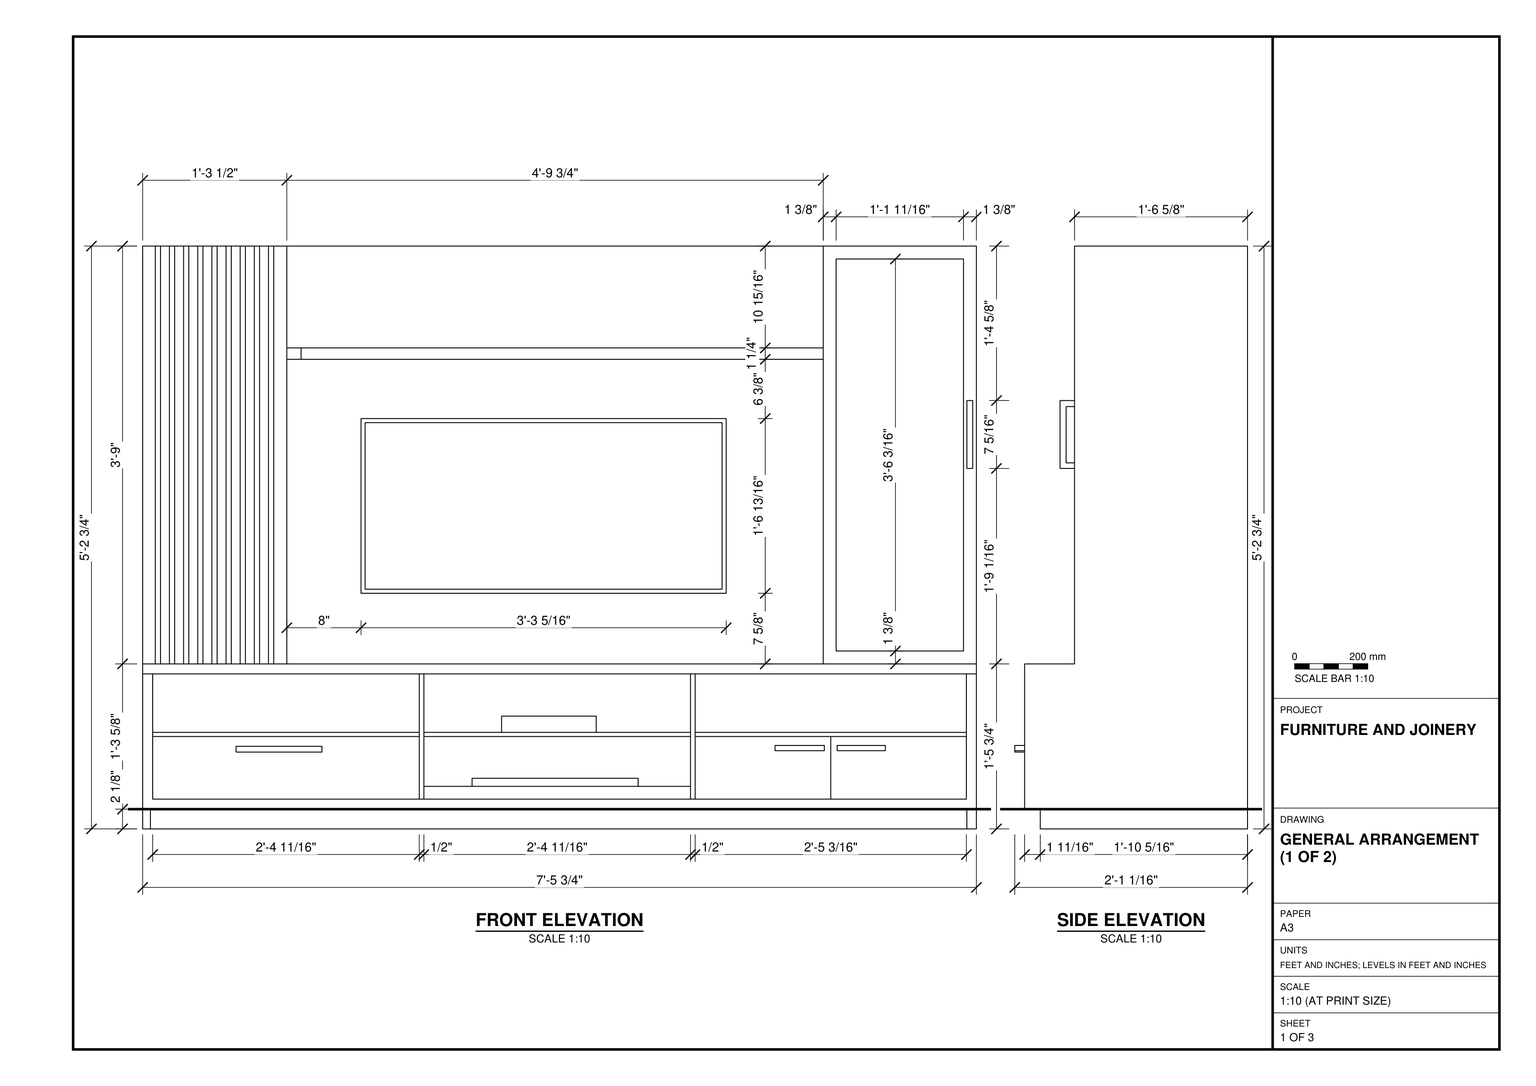
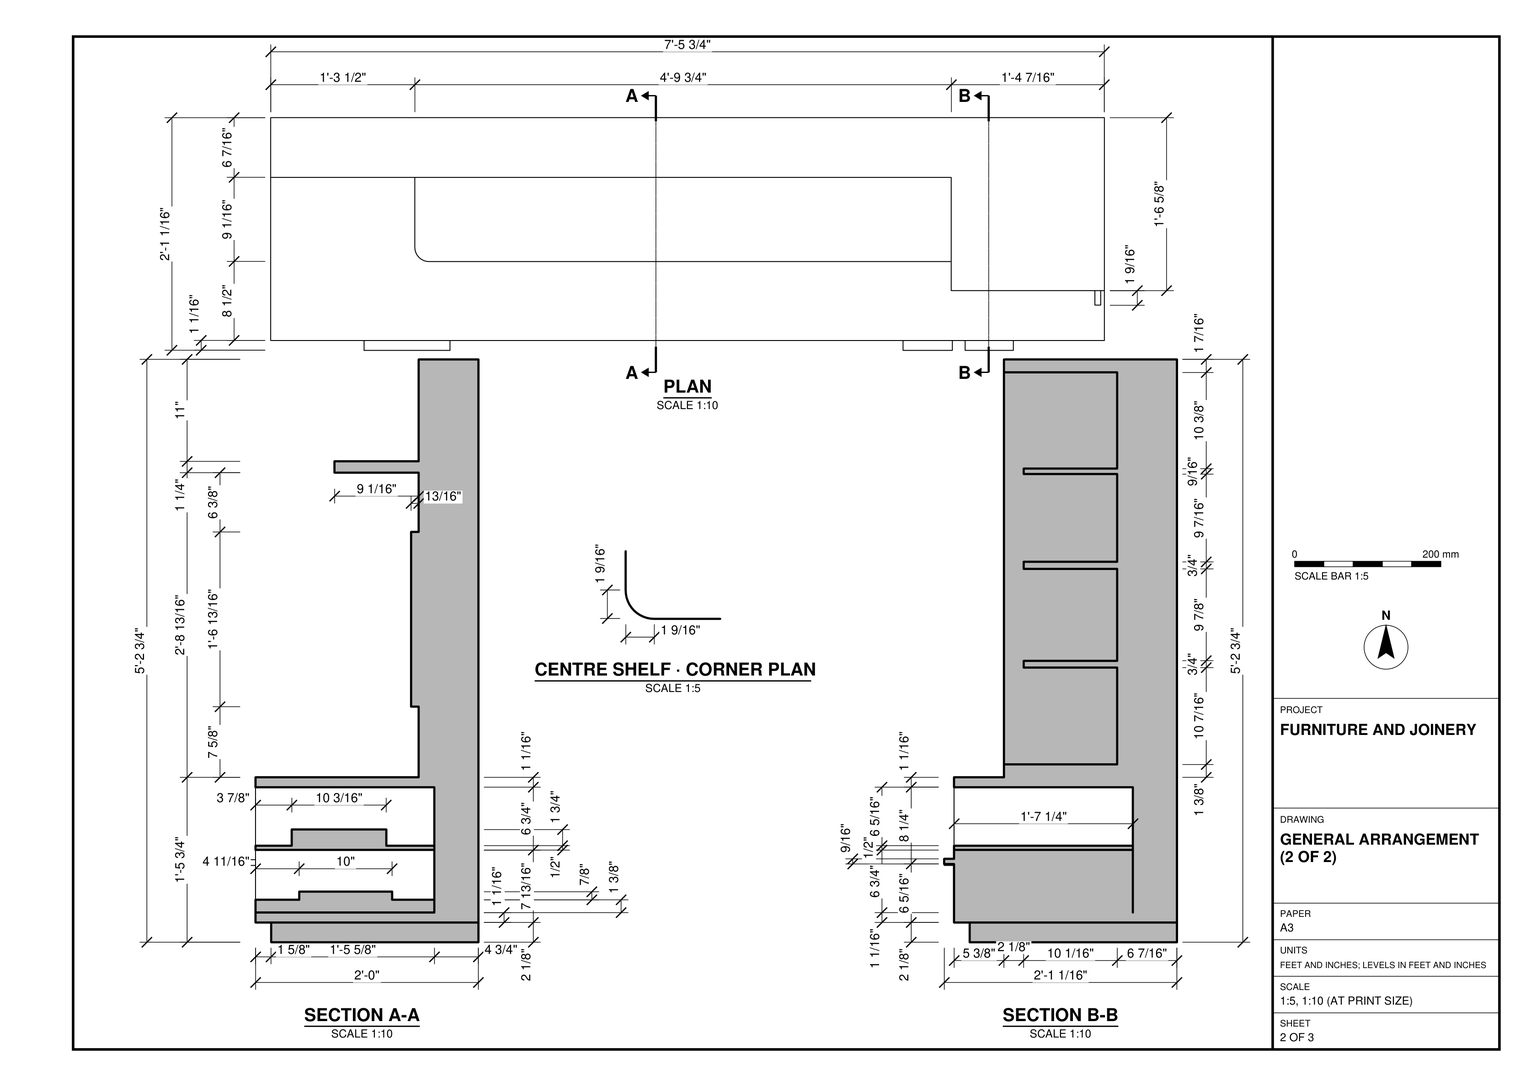
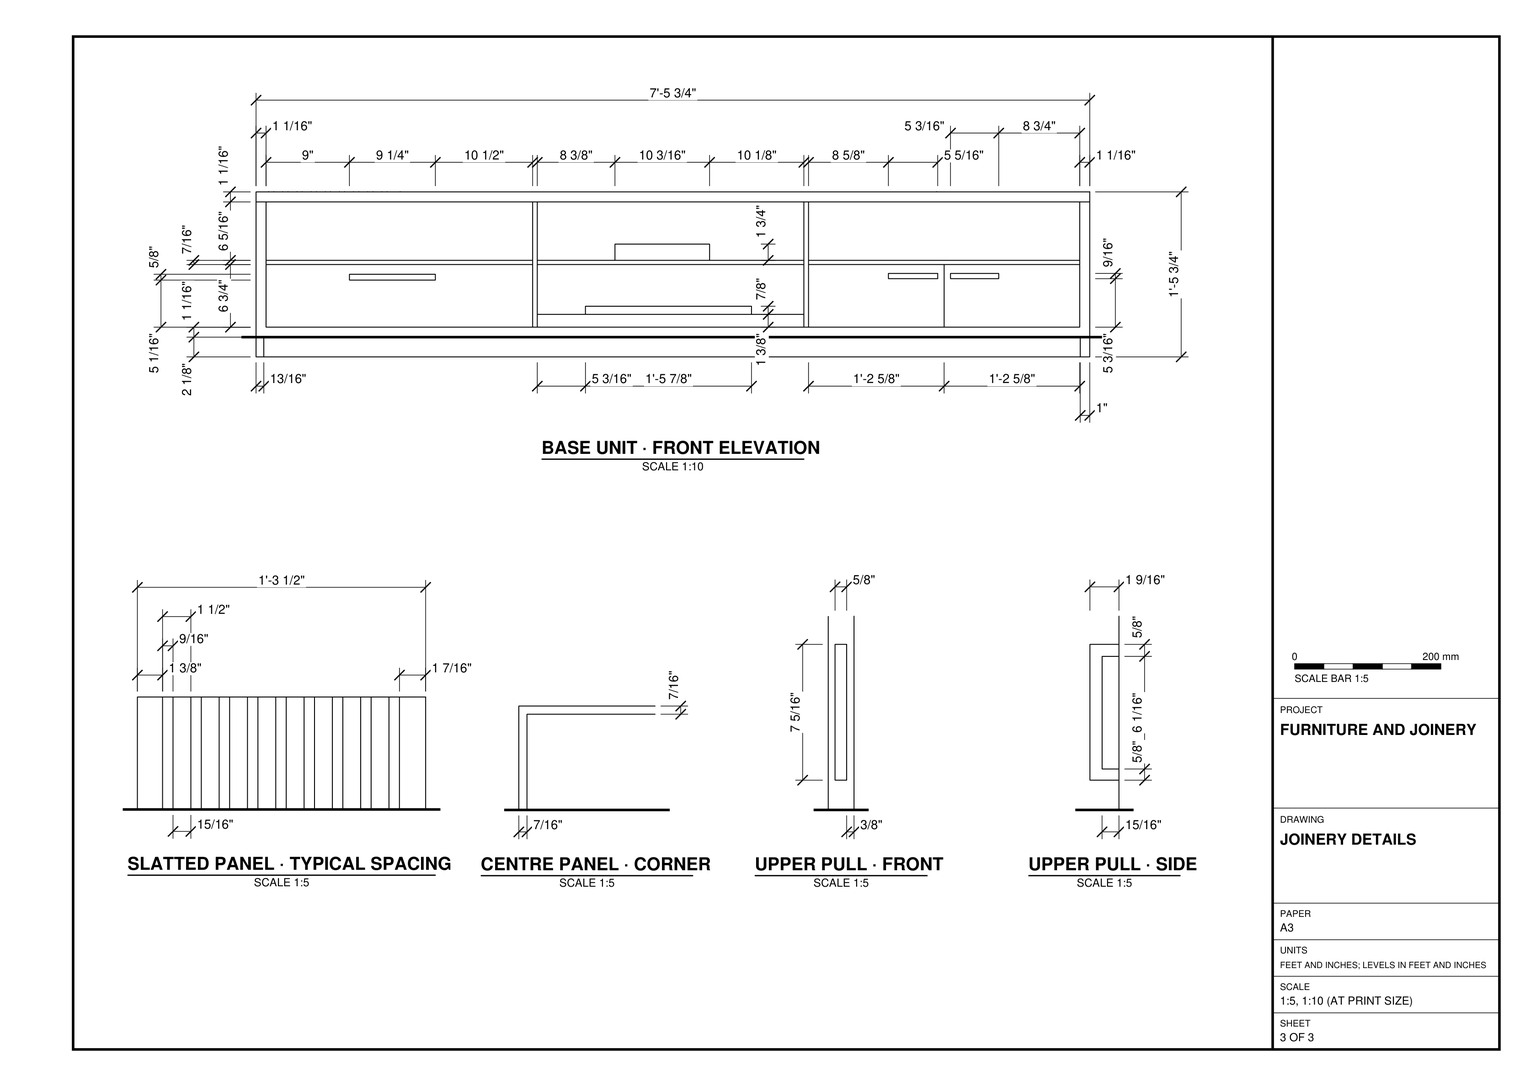
Build the media unit in SketchUp from task_files/diagram_01.pdf. Work in feet and inches, with the underside of the plinth at ±0'-0". The complete unit, including projecting pulls, is 7'-5 3/4" wide, 2'-1 1/16" deep and 5'-2 3/4" high.

Use the front elevation to lay out the low base cabinet and the three distinct areas above it. Set the base on a recessed plinth. Run its top across all three bays, with open shelving above a single lower front on the left, open shelves in the middle and paired lower fronts on the right. Fit the horizontal pulls where shown.

Above the base, form the vertical slatted panel on the left and the broad backing panel in the middle. Position the rectangular framed panel below the projecting shelf, and round the shelf's exposed front-left corner as shown in plan. Build the tall right-hand cabinet with its framed front, vertical pull and internal shelves. Use the sections to set the shelf depths, board thicknesses and setbacks rather than making the upper parts flush with the base front.

Keep the joinery parts in separate groups or components and use components for repeated parts such as slats and pulls. Decor and loose items may be any suitable library components. Save one SketchUp model as output_files/media_unit_with_a_slatted_panel_and_display_cabinet.skp.

# SketchUp Ruby script. Lengths in inches.
U = 1.inch
M = Sketchup.active_model
def pt(a) = Geom::Point3d.new(a.map { |v| v * U })
def face(e, loops, mat)
  f = e.add_face(loops[0].map { |a| pt(a) })
  loops[1..].each { |l| e.add_face(l.map { |a| pt(a) }).erase! }
  f.material = f.back_material = mat if mat
  f
end
# faces: each face lists its corners as indices into pts; further lists are holes
def faces(e, pts, list, mat = nil) = list.each { |f| face(e, (f[0].is_a?(Array) ? f : [f]).map { |l| l.map { |i| pts[i] } }, mat) }
# xy, xz, yz: faces in a plane at the given z, y or x. An outline is a flat list of corners, or four numbers for a rectangle; further outlines are holes
def ring(l) = l.size == 4 ? [[l[0], l[1]], [l[2], l[1]], [l[2], l[3]], [l[0], l[3]]] : l.each_slice(2).to_a
def flat(e, list, mat, &to3) = list.each { |f| face(e, (f[0].is_a?(Array) ? f : [f]).map { |l| ring(l).map { |u, v| to3.(u, v) } }, mat) }
def xy(e, z, list, mat = nil) = flat(e, list, mat) { |x, y| [x, y, z] }
def xz(e, y, list, mat = nil) = flat(e, list, mat) { |x, z| [x, y, z] }
def yz(e, x, list, mat = nil) = flat(e, list, mat) { |y, z| [x, y, z] }
def lines(e, pts, list) = list.each { |a, b| e.add_line(pt(pts[a]), pt(pts[b])) }
# prism: a flat outline (further loops are holes) pulled along v
def prism(e, loops, v, mat = nil)
  f = face(e, loops, mat); d = Geom::Vector3d.new(v.map { |x| x * U })
  f.pushpull(f.normal.samedirection?(d) ? d.length : -d.length)
end
def box(e, o, s, mat = nil) = prism(e, [[o, [o[0] + s[0], o[1], o[2]], [o[0] + s[0], o[1] + s[1], o[2]], [o[0], o[1] + s[1], o[2]]]], [0, 0, s[2]], mat)
def at(x, y, z, deg = 0) = Geom::Transformation.translation(pt([x, y, z])) * Geom::Transformation.rotation(ORIGIN, Z_AXIS, deg.degrees)
def axes(o, x, y, z) = Geom::Transformation.new([*x, 0, *y, 0, *z, 0, *pt(o).to_a, 1])
def part(name) = M.definitions.add(name)
# library, detail: a bought-in or finely detailed component or shape, given as its bounding box
def library(name, o, s) = part(name).tap { |d| box(d.entities, o, s) }
def detail(e, o, s) = box(e.add_group.entities, o, s)
def put(e, d, t, mat = nil) = e.add_instance(d, t).tap { |i| i.material = mat if mat }
def group(e, t, mat = nil) = e.add_group.tap { |g| g.transformation = t; g.material = mat if mat }.entities
root = M.entities
M.materials.add("[0081_CadetBlue]").color = [95, 158, 160]
M.materials.add("[0132_LightGray]").color = [169, 169, 169]
M.materials.add("[0136_Charcoal]").color = [35, 35, 35]
M.materials.add("[0137_Black]").color = [0, 0, 0]
M.materials.add("[Translucent Glass Gray]").color = [209, 209, 209]
M.materials["[Translucent Glass Gray]"].alpha = 0.5
xy(root,7.08,[[0,2.75,89.75,25.0625]],"[0081_CadetBlue]")
xy(root,9.21,[[0,1.0625,89.75,2.75],[0,2.75,89.75,25.0625]])
xy(root,10.29,[[29.78,1.0625,30.28,20.3125],[30.28,1.0625,58.97,20.3125],[58.97,1.0625,59.47,20.3125]])
xy(root,11.66,[[[30.28,1.0625,58.97,20.3125],[35.46,5.77,53.34,15.77]]],"[0081_CadetBlue]")
xy(root,12.54,[[35.46,5.77,53.34,15.77]],"[0136_Charcoal]")
xy(root,15.35,[[10.05,0,19.3,1.0625]],"[0132_LightGray]")
xy(root,15.5,[[68.07,0,73.39,1.0625],[74.76,0,79.95,1.0625]],"[0132_LightGray]")
xy(root,15.98,[[10.05,0,19.3,1.0625]],"[0132_LightGray]")
xy(root,16.07,[[68.07,0,73.39,1.0625],[74.76,0,79.95,1.0625]],"[0132_LightGray]")
xy(root,17.03,[[1.08,1.0625,29.78,20.3125],[59.47,1.0625,88.67,20.3125]])
xy(root,17.03,[[30.28,1.0625,58.97,20.3125]],"[0081_CadetBlue]")
xy(root,17.48,[[1.08,1.0625,29.78,20.3125],[[30.28,1.0625,58.97,20.3125],[38.64,4.96,48.82,15.15]],[59.47,1.0625,88.67,20.3125]])
xy(root,19.23,[[38.64,4.96,48.82,15.15]],"[0136_Charcoal]")
xy(root,23.77,[[1.08,1.0625,29.78,20.3125],[29.78,1.0625,30.28,20.3125],[30.28,1.0625,58.97,20.3125],[58.97,1.0625,59.47,20.3125],[59.47,1.0625,88.67,20.3125]])
xy(root,24.85,[[0,1.0625,89.75,1.0625,89.75,6.4375,73.26,6.4375,73.26,18.625,0,18.625]])
xy(root,26.24,[[74.65,6.4375,88.36,18.625]])
xy(root,32.45,[[23.5,17.8125,62.82,18.625]],"[0137_Black]")
xy(root,36.66,[[74.65,8.5625,88.36,18.625]])
xy(root,37.38,[[74.65,8.5625,88.36,18.625]])
xy(root,45.89,[[88.73,4.875,89.35,6.4375]])
xy(root,46.49,[[88.73,5.53,89.35,6.4375]])
xy(root,47.28,[[74.65,8.5625,88.36,18.625]])
xy(root,48.05,[[74.65,8.5625,88.36,18.625]])
xy(root,51.26,[[23.5,17.8125,62.82,18.625]],"[0137_Black]")
xy(root,52.56,[[88.73,5.53,89.35,6.4375]])
xy(root,53.21,[[88.73,4.875,89.35,6.4375]])
xy(root,57.5,[[74.65,8.5625,88.36,18.625]])
xy(root,57.64,[[17.05,9.5625,16.85,9.58,16.66,9.61,16.47,9.68,16.29,9.77,16.12,9.88,15.97,10.01,15.83,10.16,15.72,10.33,15.63,10.51,15.57,10.7,15.53,10.9,15.52,11.1,15.52,18.625,73.26,18.625,73.26,9.5625]])
xy(root,58.09,[[74.65,8.5625,88.36,18.625]])
xy(root,58.87,[[17.05,9.5625,73.26,9.5625,73.26,18.625,15.52,18.625,15.52,11.1,15.53,10.9,15.57,10.7,15.63,10.51,15.72,10.33,15.83,10.16,15.97,10.01,16.12,9.88,16.29,9.77,16.47,9.68,16.66,9.61,16.85,9.58]],"[0081_CadetBlue]")
xy(root,68.45,[[74.65,6.4375,88.36,18.625]])
xy(root,69.83,[[73.26,6.4375,89.75,6.4375,89.75,25.0625,0,25.0625,0,18.625,73.26,18.625]],"[0081_CadetBlue]")
xz(root,0,[[10.05,15.35,19.3,15.98],[68.07,15.5,73.39,16.07],[74.76,15.5,79.95,16.07]],"[0132_LightGray]")
xz(root,1.0625,[[[1.08,10.29,29.78,17.03],[10.05,15.35,19.3,15.98]],[[59.47,10.29,74.07,17.03],[68.07,15.5,73.39,16.07]],[[74.07,10.29,88.67,17.03],[74.76,15.5,79.95,16.07]],[1.08,17.03,29.78,17.48],[59.47,17.03,88.67,17.48],
  [0,23.77,89.75,24.85]])
xz(root,1.0625,[[0,9.21,89.75,9.21,89.75,23.77,88.67,23.77,88.67,10.29,1.08,10.29,1.08,23.77,0,23.77],[29.78,10.29,30.28,23.77],[30.28,10.29,58.97,11.66],[58.97,10.29,59.47,23.77],[30.28,17.03,58.97,17.48]],"[0081_CadetBlue]")
xz(root,2.75,[[0,7.08,0.84,9.21],[0.84,7.08,88.72,9.21],[88.72,7.08,89.75,9.21]],"[0081_CadetBlue]")
xz(root,4.875,[[88.73,45.89,89.35,53.21]],"[0137_Black]")
xz(root,4.96,[[38.64,17.48,48.82,19.23]],"[0136_Charcoal]")
xz(root,5.53,[[88.73,46.49,89.35,52.56]])
xz(root,5.77,[[35.46,11.66,53.34,12.54]],"[0136_Charcoal]")
xz(root,6.4375,[[[73.26,24.85,89.75,69.83],[74.65,26.24,88.36,68.45],[88.73,52.56,89.35,53.21],[88.73,45.89,89.35,46.49]]],"[0081_CadetBlue]")
xz(root,6.4375,[[74.65,26.24,88.36,68.45]],"[Translucent Glass Gray]")
xz(root,8.5625,[[74.65,36.66,88.36,37.38],[74.65,47.28,88.36,48.05],[74.65,57.5,88.36,58.09]])
xz(root,9.5625,[[17.05,57.64,73.26,58.87]],"[0081_CadetBlue]")
xz(root,15.15,[[38.64,17.48,48.82,19.23]])
xz(root,15.77,[[35.46,11.66,53.34,12.54]])
xz(root,17.8125,[[[23.5,32.45,62.82,51.26],[23.94,32.89,62.375,50.82]],[23.94,32.89,62.375,50.82]],"[0137_Black]")
xz(root,18.625,[[1.36,24.85,1.92,69.83],[2.88,24.85,3.44,69.83],[4.4,24.85,4.97,69.83],[5.93,24.85,6.49,69.83],[7.45,24.85,8.01,69.83],
  [8.97,24.85,9.54,69.83],[10.5,24.85,11.06,69.83],[12.02,24.85,12.58,69.83],[13.54,24.85,14.11,69.83],[[15.52,24.85,73.26,57.64],[23.5,32.45,62.82,51.26]],
  [74.65,26.24,88.36,36.66],[74.65,37.38,88.36,47.28],[74.65,48.05,88.36,57.5],[74.65,58.09,88.36,68.45],[15.52,58.87,73.26,69.83]])
xz(root,18.625,[[0,24.85,1.36,69.83],[1.92,24.85,2.88,69.83],[3.44,24.85,4.4,69.83],[4.97,24.85,5.93,69.83],[6.49,24.85,7.45,69.83],
  [8.01,24.85,8.97,69.83],[9.54,24.85,10.5,69.83],[11.06,24.85,12.02,69.83],[12.58,24.85,13.54,69.83],[14.11,24.85,15.52,69.83]],"[0081_CadetBlue]")
xz(root,20.3125,[[1.08,10.29,29.78,17.03],[29.78,10.29,30.28,23.77],[30.28,10.29,58.97,11.66],[58.97,10.29,59.47,23.77],[59.47,10.29,88.67,17.03],
  [30.28,11.66,58.97,17.03],[1.08,17.03,29.78,17.48],[30.28,17.03,58.97,17.48],[59.47,17.03,88.67,17.48],[1.08,17.48,29.78,23.77],
  [30.28,17.48,58.97,23.77],[59.47,17.48,88.67,23.77]])
xz(root,25.0625,[[0,7.08,89.75,9.21],[0,9.21,89.75,69.83]],"[0081_CadetBlue]")
yz(root,0,[[2.75,7.08,25.0625,9.21],[1.0625,9.21,1.0625,24.85,18.625,24.85,18.625,69.83,25.0625,69.83,25.0625,9.21]],"[0081_CadetBlue]")
yz(root,1.08,[[1.0625,10.29,20.3125,17.03],[1.0625,17.03,20.3125,17.48]])
yz(root,1.08,[[1.0625,17.48,20.3125,23.77]],"[0081_CadetBlue]")
yz(root,10.05,[[0,15.35,1.0625,15.98]],"[0132_LightGray]")
yz(root,15.52,[[11.1,57.64,18.625,58.87]],"[0081_CadetBlue]")
yz(root,19.3,[[0,15.35,1.0625,15.98]],"[0132_LightGray]")
yz(root,23.5,[[17.8125,32.45,18.625,51.26]],"[0137_Black]")
yz(root,29.78,[[1.0625,10.29,20.3125,17.03],[1.0625,17.03,20.3125,17.48]])
yz(root,29.78,[[1.0625,17.48,20.3125,23.77]],"[0081_CadetBlue]")
yz(root,30.28,[[1.0625,10.29,20.3125,11.66],[1.0625,17.03,20.3125,17.48]])
yz(root,30.28,[[1.0625,11.66,20.3125,17.03],[1.0625,17.48,20.3125,23.77]],"[0081_CadetBlue]")
yz(root,35.46,[[5.77,11.66,15.77,12.54]],"[0136_Charcoal]")
yz(root,38.64,[[4.96,17.48,15.15,19.23]],"[0136_Charcoal]")
yz(root,48.82,[[4.96,17.48,15.15,19.23]],"[0136_Charcoal]")
yz(root,53.34,[[5.77,11.66,15.77,12.54]],"[0136_Charcoal]")
yz(root,58.97,[[1.0625,10.29,20.3125,11.66],[1.0625,17.03,20.3125,17.48]])
yz(root,58.97,[[1.0625,11.66,20.3125,17.03],[1.0625,17.48,20.3125,23.77]],"[0081_CadetBlue]")
yz(root,59.47,[[1.0625,10.29,20.3125,17.03],[1.0625,17.03,20.3125,17.48]])
yz(root,59.47,[[1.0625,17.48,20.3125,23.77]],"[0081_CadetBlue]")
yz(root,62.82,[[17.8125,32.45,18.625,51.26]],"[0137_Black]")
yz(root,68.07,[[0,15.5,1.0625,16.07]],"[0132_LightGray]")
yz(root,73.26,[[6.4375,24.85,6.4375,69.83,18.625,69.83,18.625,58.87,9.5625,58.87,9.5625,57.64,18.625,57.64,18.625,24.85]],"[0081_CadetBlue]")
yz(root,73.39,[[0,15.5,1.0625,16.07]])
yz(root,74.65,[[6.4375,26.24,18.625,26.24,18.625,36.66,8.5625,36.66,8.5625,37.38,18.625,37.38,18.625,47.28,8.5625,47.28,8.5625,48.05,18.625,48.05,18.625,57.5,8.5625,57.5,8.5625,58.09,18.625,58.09,18.625,68.45,6.4375,68.45]])
yz(root,74.76,[[0,15.5,1.0625,16.07]],"[0132_LightGray]")
yz(root,79.95,[[0,15.5,1.0625,16.07]])
yz(root,88.36,[[6.4375,26.24,6.4375,68.45,18.625,68.45,18.625,58.09,8.5625,58.09,8.5625,57.5,18.625,57.5,18.625,48.05,8.5625,48.05,8.5625,47.28,18.625,47.28,18.625,37.38,8.5625,37.38,8.5625,36.66,18.625,36.66,18.625,26.24]])
yz(root,88.67,[[1.0625,10.29,20.3125,17.03],[1.0625,17.03,20.3125,17.48]])
yz(root,88.67,[[1.0625,17.48,20.3125,23.77]],"[0081_CadetBlue]")
yz(root,88.73,[[4.875,45.89,4.875,53.21,6.4375,53.21,6.4375,52.56,5.53,52.56,5.53,46.49,6.4375,46.49,6.4375,45.89]],"[0137_Black]")
yz(root,89.35,[[4.875,45.89,6.4375,45.89,6.4375,46.49,5.53,46.49,5.53,52.56,6.4375,52.56,6.4375,53.21,4.875,53.21]],"[0137_Black]")
yz(root,89.75,[[2.75,7.08,25.0625,9.21],[1.0625,9.21,25.0625,9.21,25.0625,69.83,6.4375,69.83,6.4375,24.85,1.0625,24.85]],"[0081_CadetBlue]")
p = [[16.66,9.61,58.87],[16.47,9.68,58.87],[16.47,9.68,57.64],[16.66,9.61,57.64],[16.85,9.58,58.87],[16.85,9.58,57.64],
  [17.05,9.5625,58.87],[17.05,9.5625,57.64],[16.29,9.77,58.87],[16.29,9.77,57.64],[16.12,9.88,58.87],[16.12,9.88,57.64],
  [15.97,10.01,58.87],[15.97,10.01,57.64],[15.83,10.16,58.87],[15.83,10.16,57.64],[15.72,10.33,58.87],[15.72,10.33,57.64],
  [15.63,10.51,58.87],[15.63,10.51,57.64],[15.57,10.7,58.87],[15.57,10.7,57.64],[15.53,10.9,58.87],[15.53,10.9,57.64],
  [15.52,11.1,58.87],[15.52,11.1,57.64]]
faces(root,p,[[0,1,2,3],[4,0,3,5],[6,4,5,7],[1,8,9,2],[8,10,11,9],[10,12,13,11],[12,14,15,13],[14,16,17,15],
  [16,18,19,17],[18,20,21,19],[20,22,23,21],[22,24,25,23]],"[0081_CadetBlue]")
